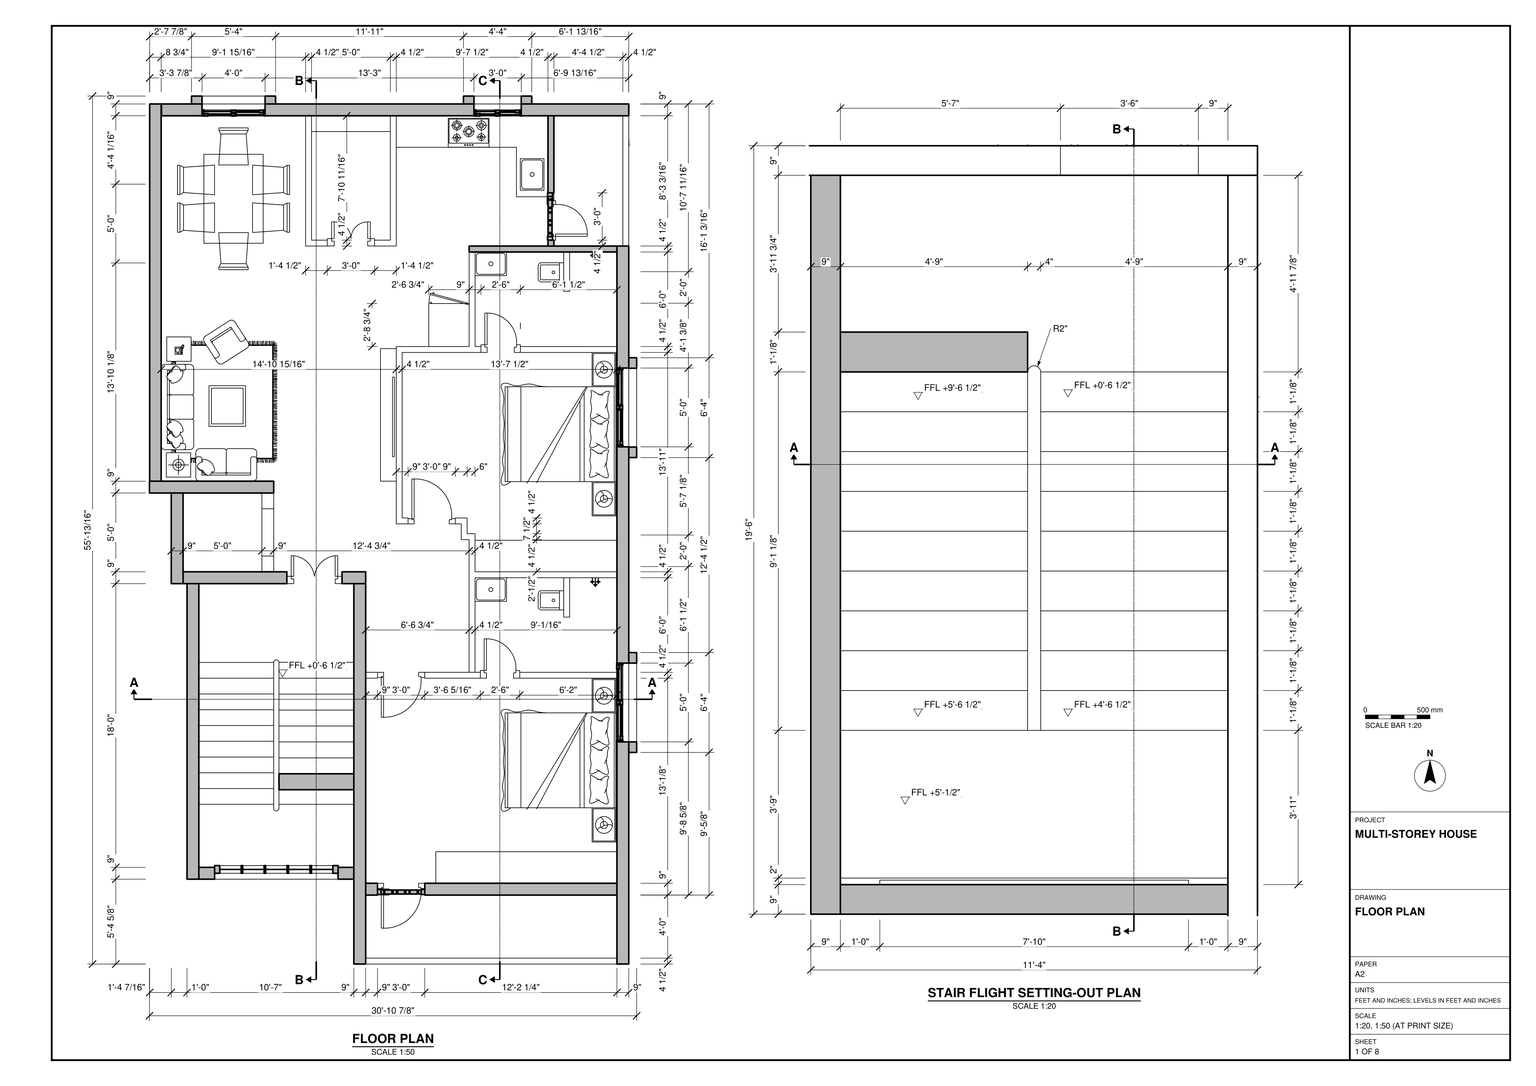
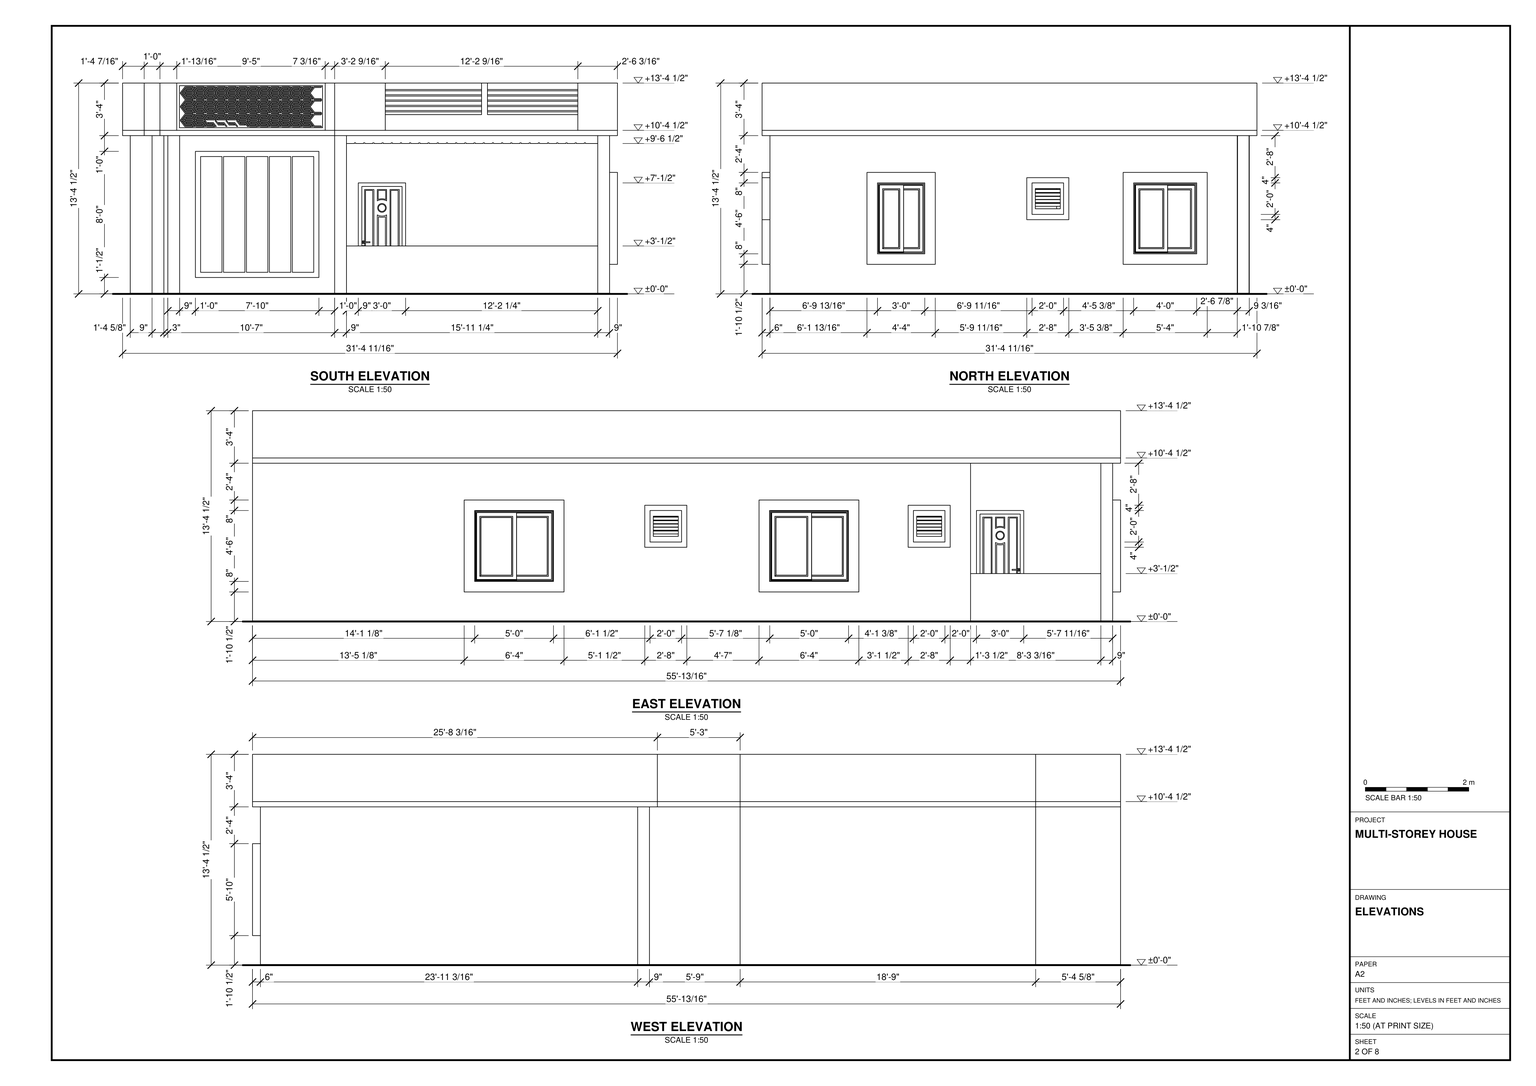
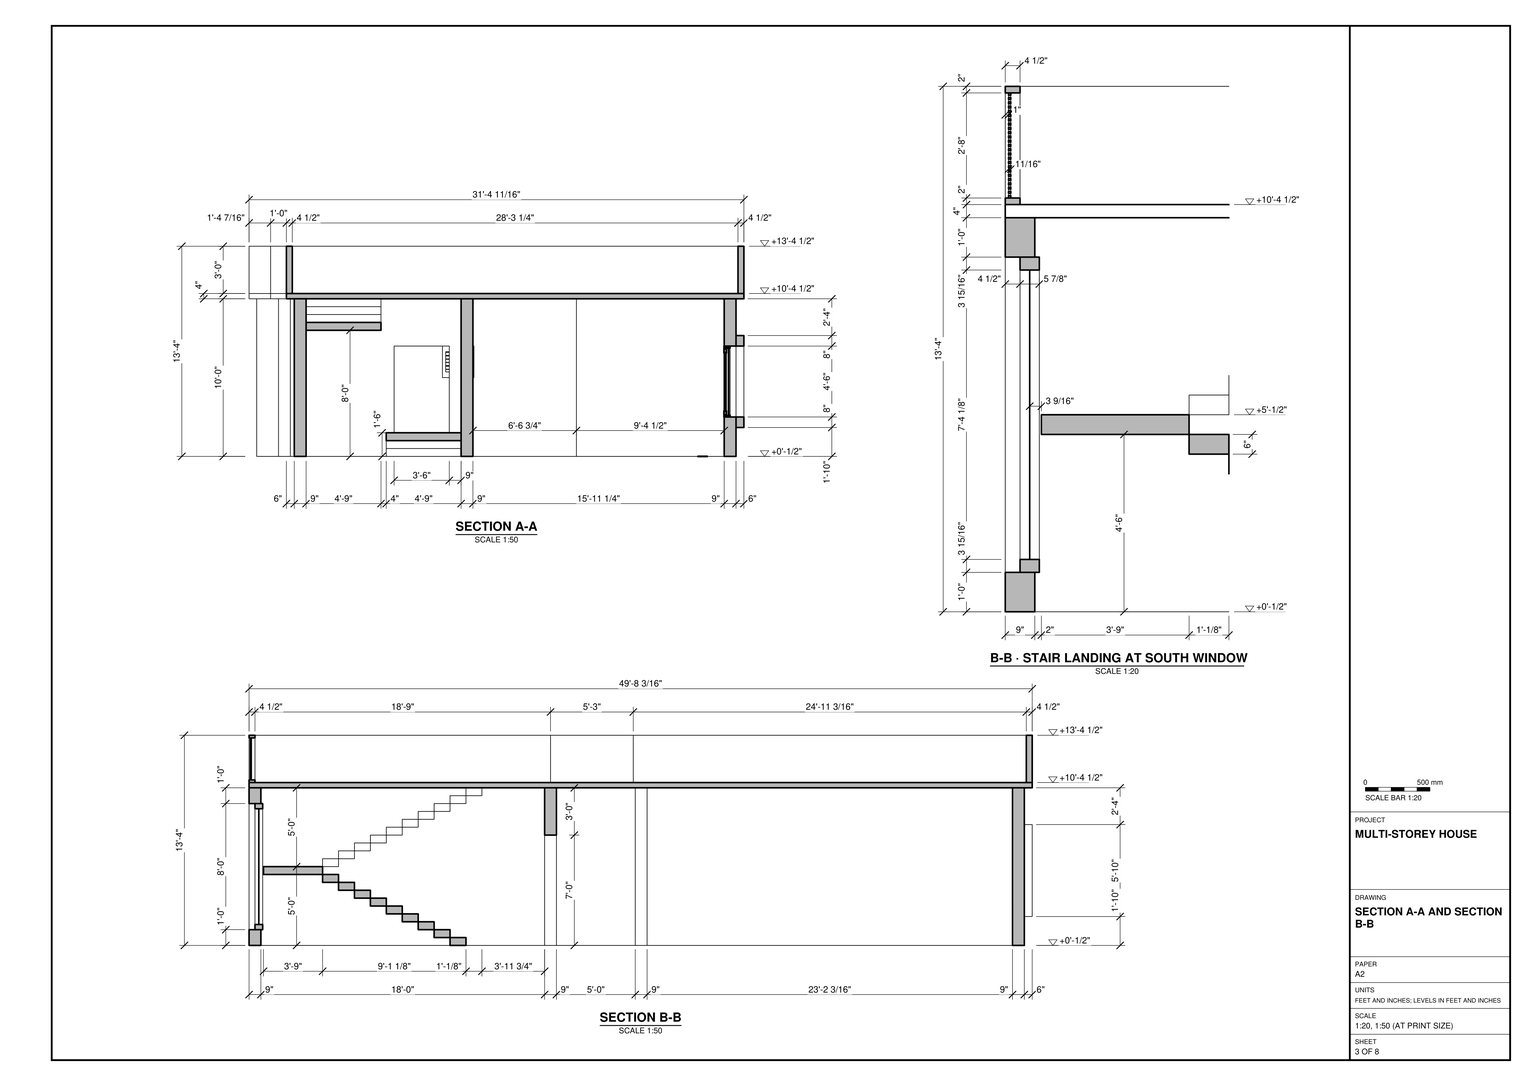
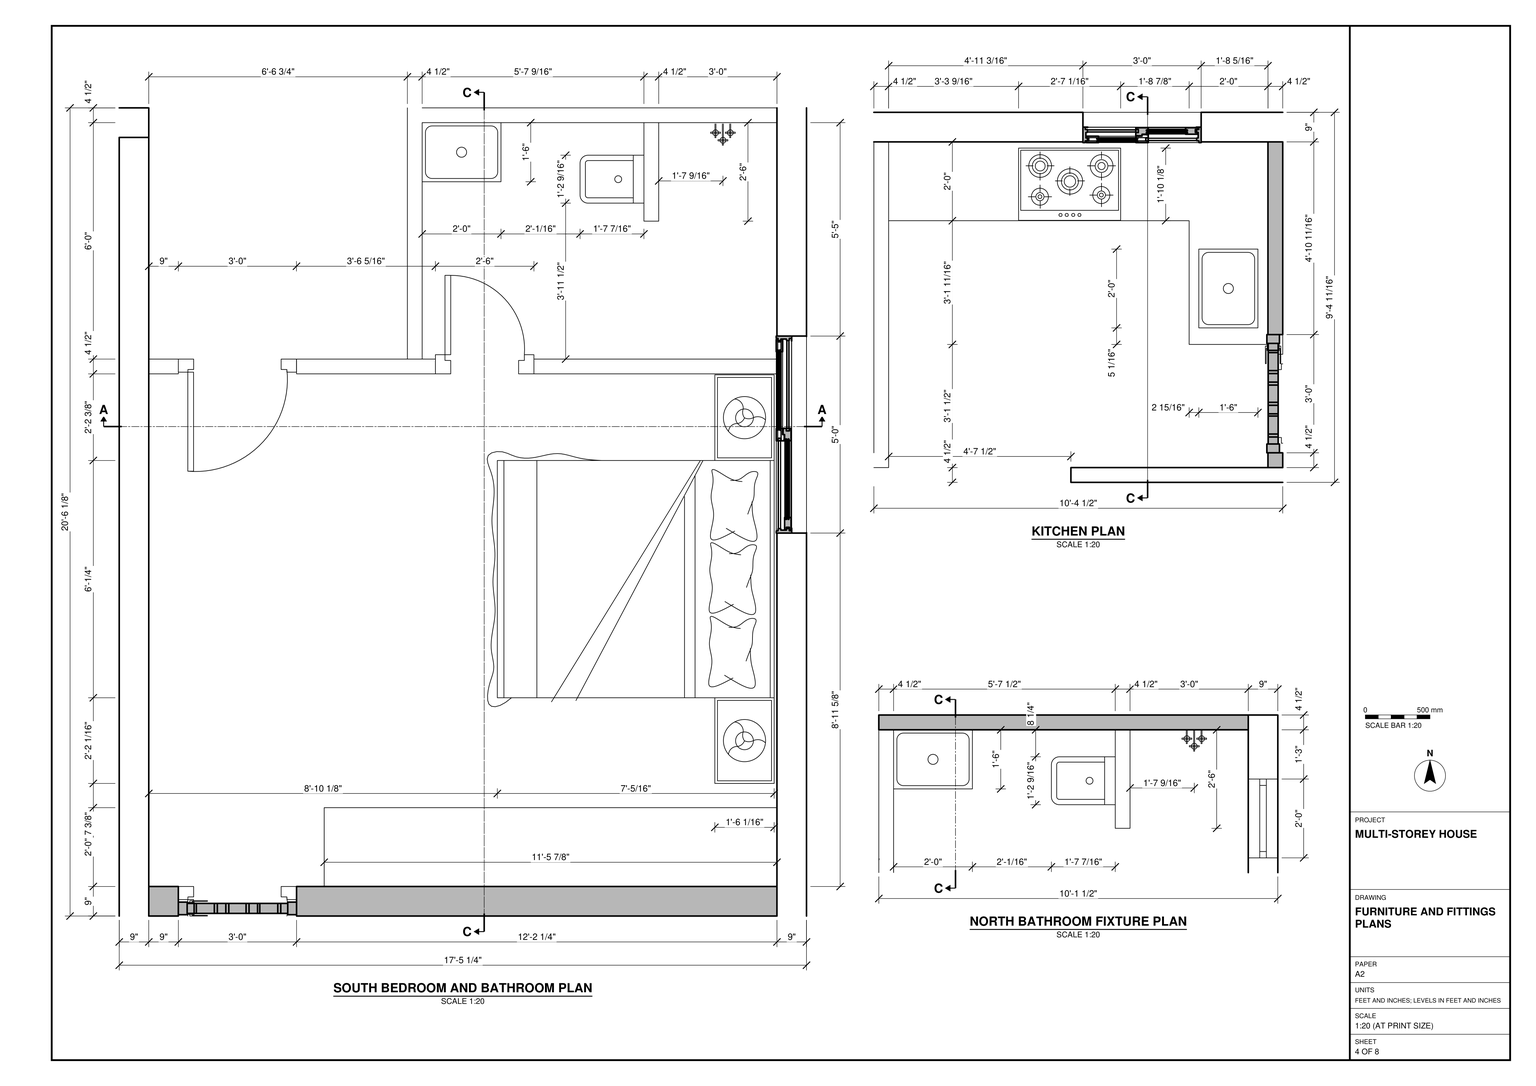
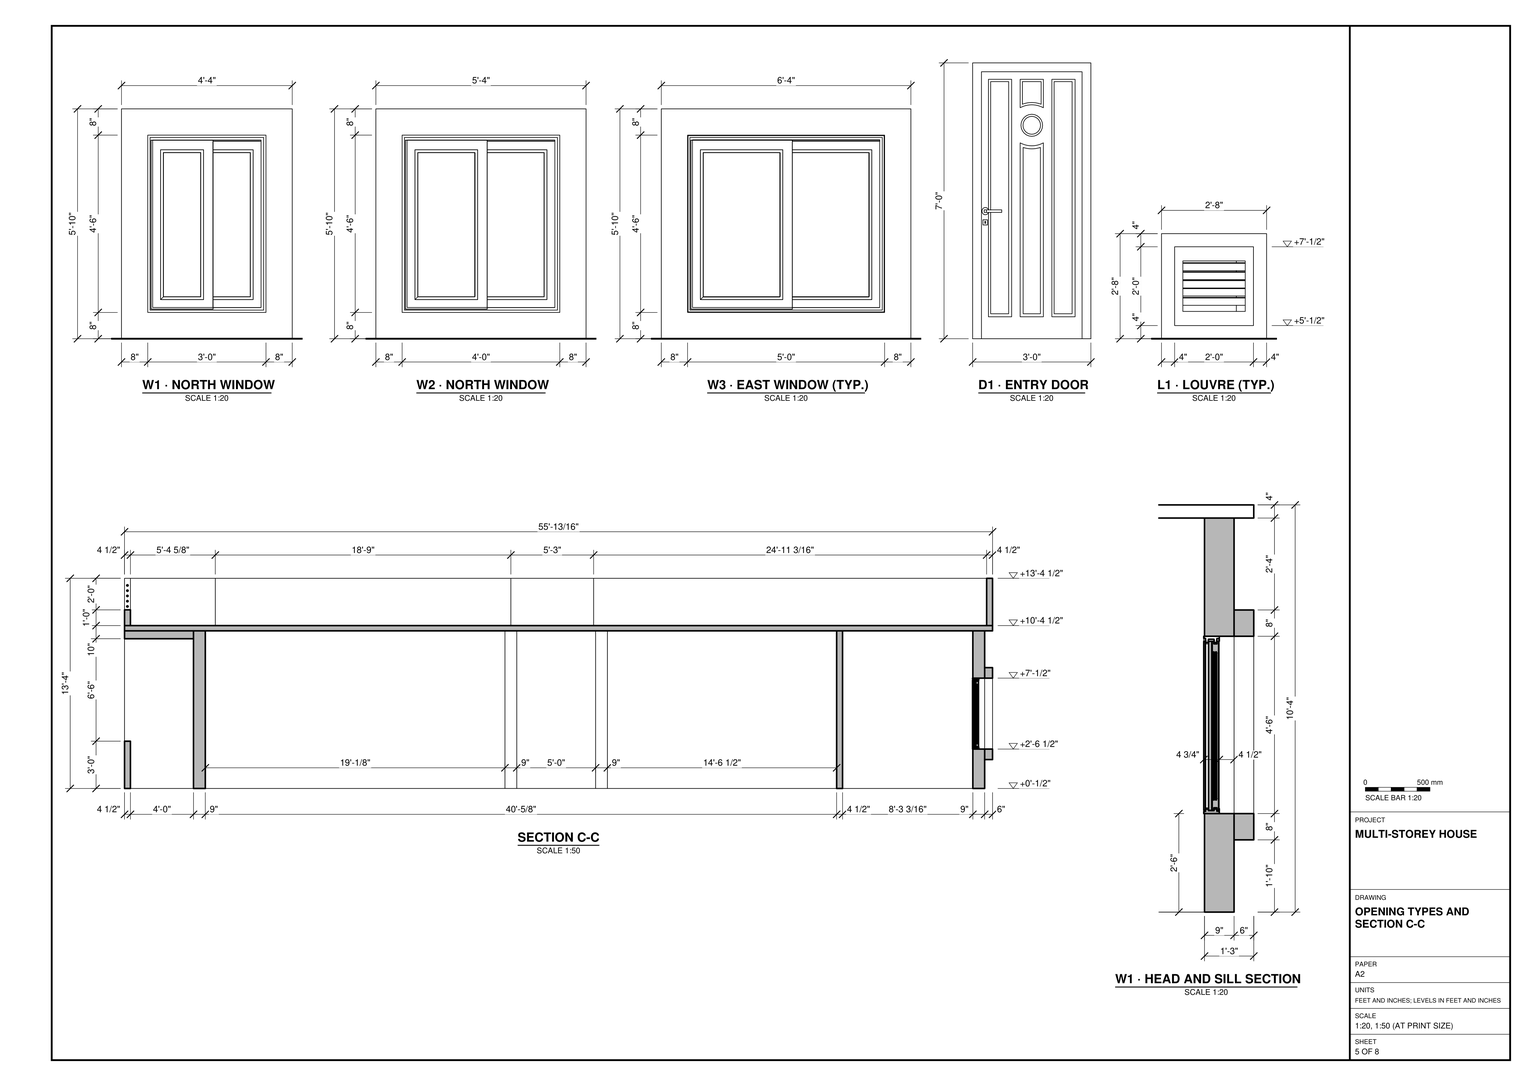
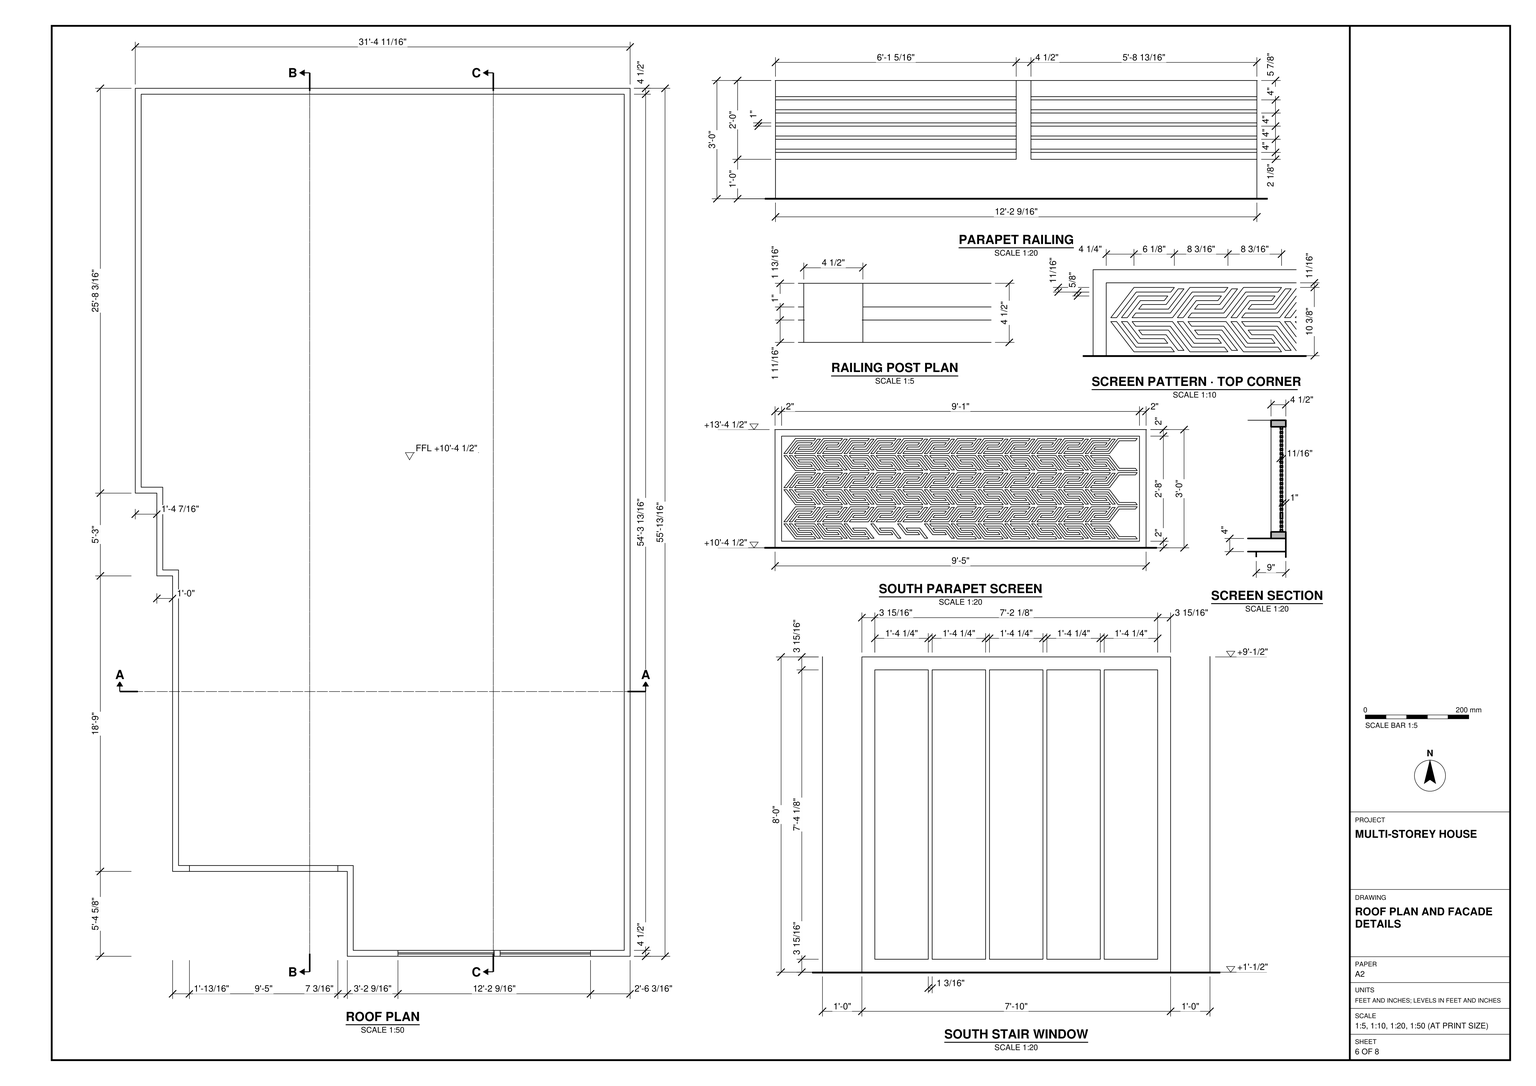
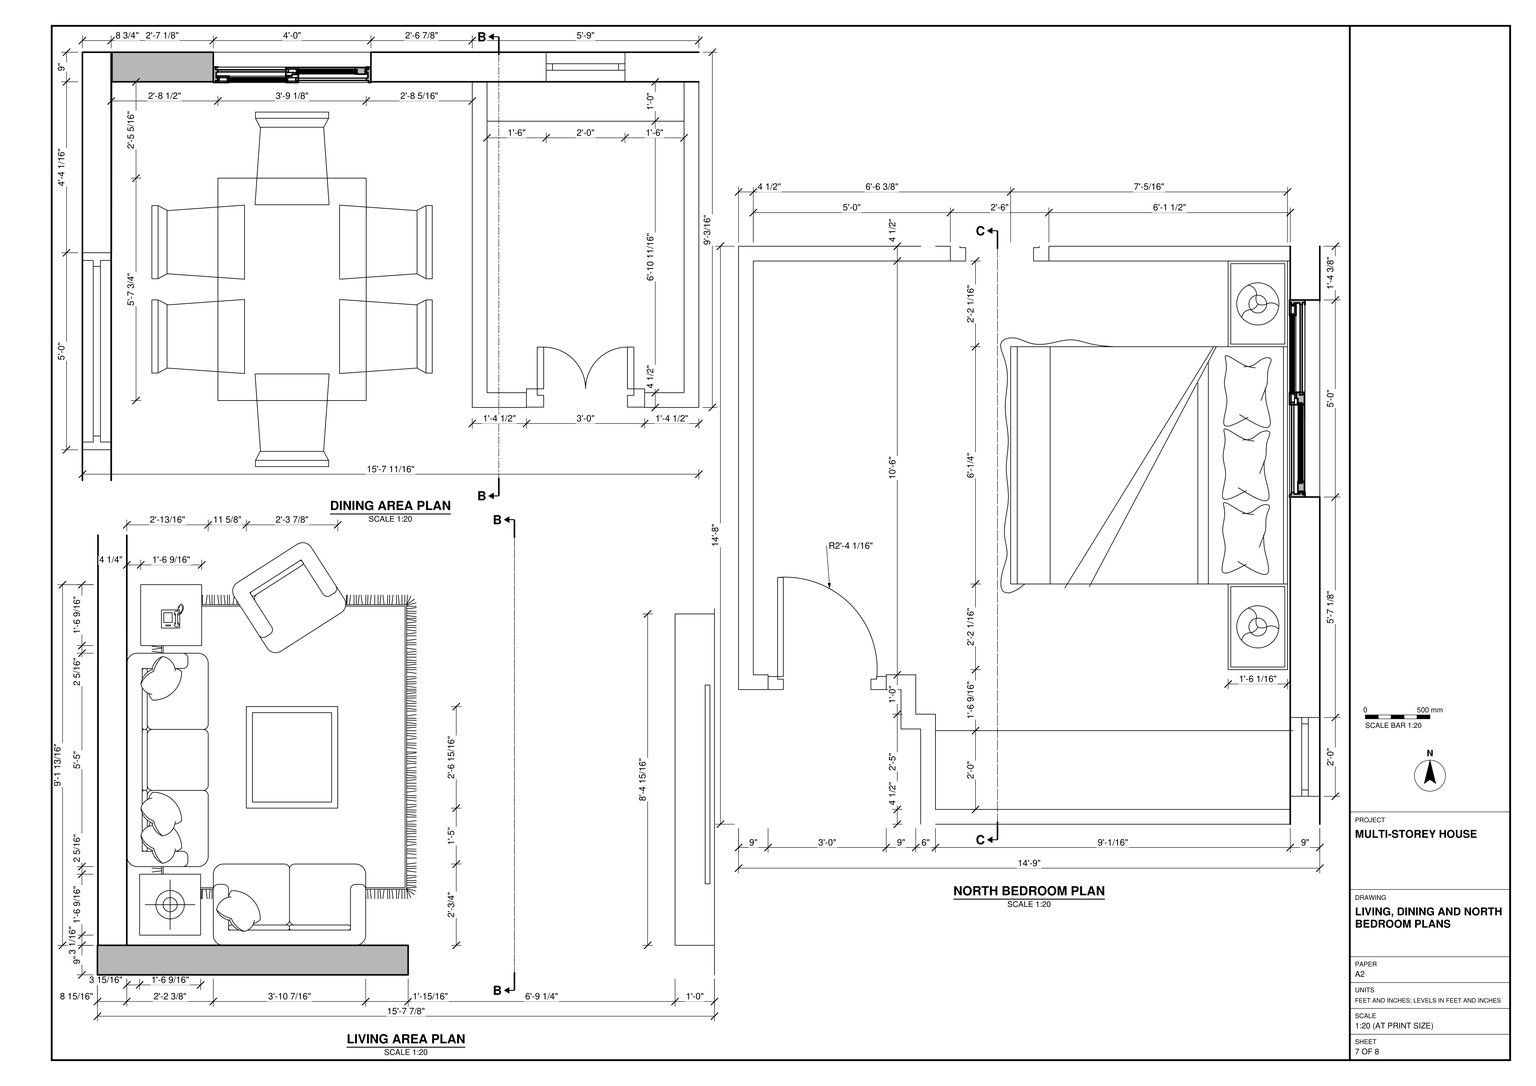
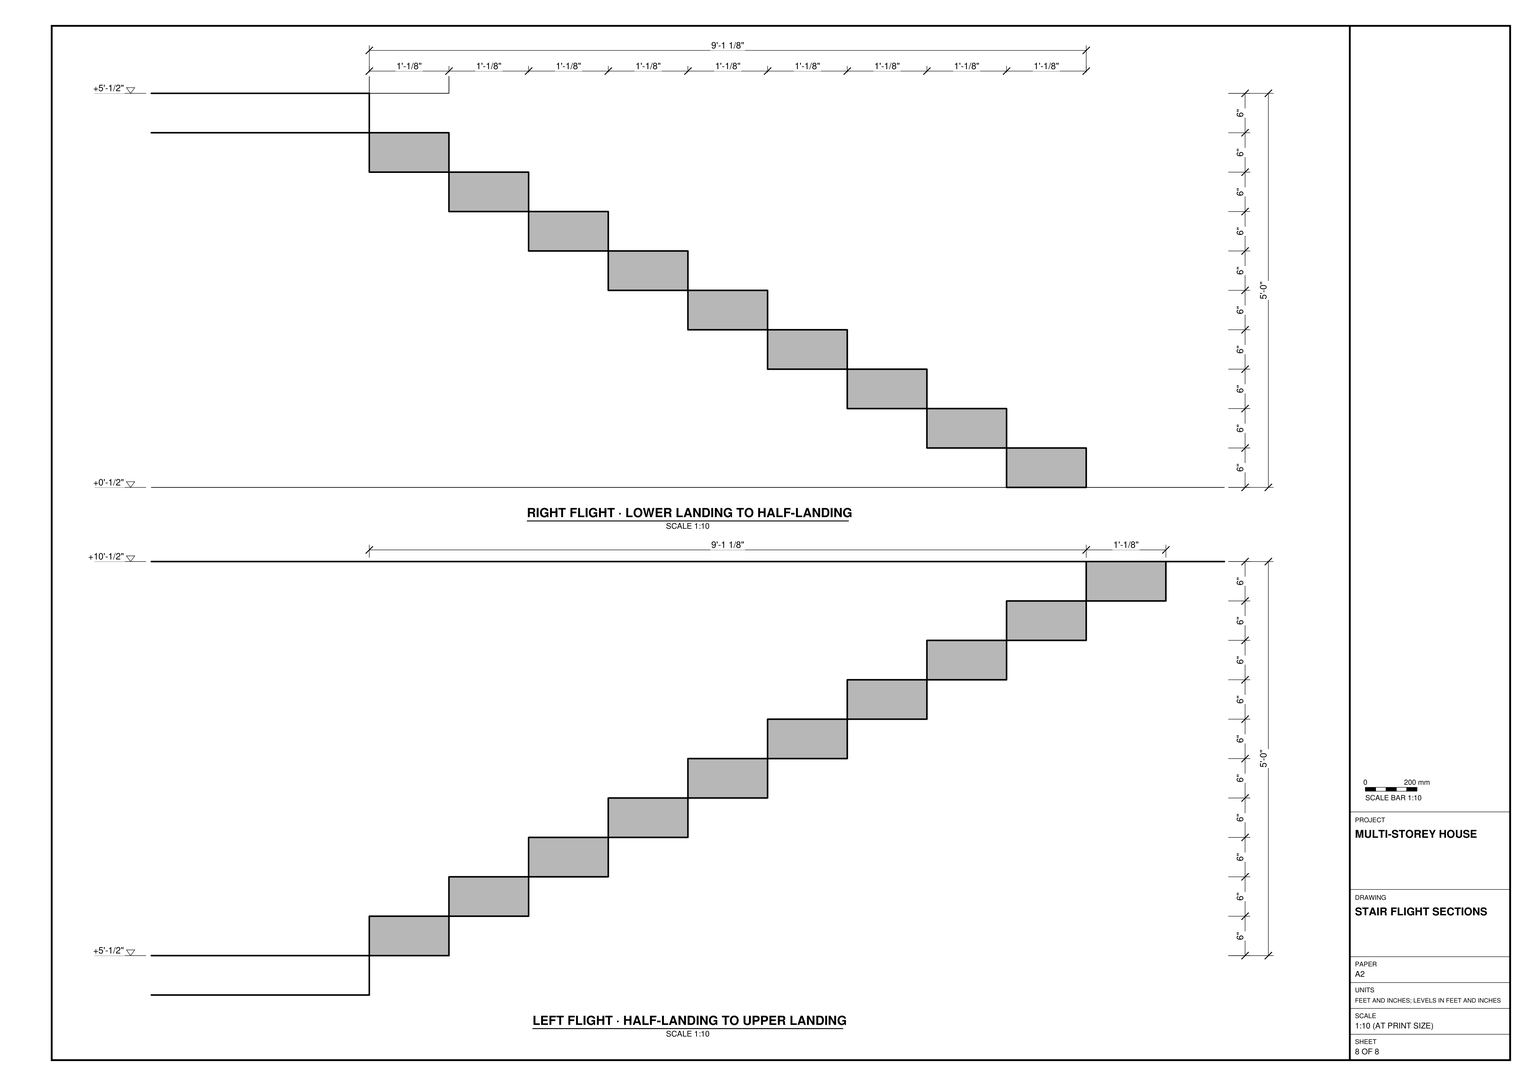
Build the house in SketchUp from task_files/diagram_01.pdf. Work in feet and inches. Set the ground-floor datum to ±0'-0". The overall dimensions, including exterior projections, are 31'-4 11/16" along X, 55'-13/16" along Y and 13'-4 1/2" in height.

Follow the floor plan for the stepped footprint, recessed entrance and room connections. Place the living and dining areas on the west side, the kitchen at the north end and the two bedrooms and adjoining bathrooms along the east side. Use the wall thicknesses shown, distinguishing the 9" walls from the 4 1/2" partitions. Model the floor slab, doors, framed windows and ventilators. Use the stair setting-out plan and sections to build the two parallel flights and their connecting landing at the tall south window. Model the flat roof slab and parapet, including the perforated screen and horizontal slats on the south elevation.

Fit the kitchen counters, sink and cooktop to the plan. Include the bathroom fixtures, beds, bedside tables, living room seating and dining furniture at the sizes and positions drawn. Decor and loose items may be any suitable library components. Keep shell elements such as walls, slabs and roof, and each furniture or joinery piece, as separate groups or components; use components for repeated parts. Save one SketchUp model as output_files/two_bedroom_house_with_a_return_stair_and_flat_roof.skp.

# SketchUp Ruby script. Lengths in inches.
U = 1.inch
M = Sketchup.active_model
def pt(a) = Geom::Point3d.new(a.map { |v| v * U })
def face(e, loops, mat)
  f = e.add_face(loops[0].map { |a| pt(a) })
  loops[1..].each { |l| e.add_face(l.map { |a| pt(a) }).erase! }
  f.material = f.back_material = mat if mat
  f
end
# faces: each face lists its corners as indices into pts; further lists are holes
def faces(e, pts, list, mat = nil) = list.each { |f| face(e, (f[0].is_a?(Array) ? f : [f]).map { |l| l.map { |i| pts[i] } }, mat) }
# xy, xz, yz: faces in a plane at the given z, y or x. An outline is a flat list of corners, or four numbers for a rectangle; further outlines are holes
def ring(l) = l.size == 4 ? [[l[0], l[1]], [l[2], l[1]], [l[2], l[3]], [l[0], l[3]]] : l.each_slice(2).to_a
def flat(e, list, mat, &to3) = list.each { |f| face(e, (f[0].is_a?(Array) ? f : [f]).map { |l| ring(l).map { |u, v| to3.(u, v) } }, mat) }
def xy(e, z, list, mat = nil) = flat(e, list, mat) { |x, y| [x, y, z] }
def xz(e, y, list, mat = nil) = flat(e, list, mat) { |x, z| [x, y, z] }
def yz(e, x, list, mat = nil) = flat(e, list, mat) { |y, z| [x, y, z] }
def lines(e, pts, list) = list.each { |a, b| e.add_line(pt(pts[a]), pt(pts[b])) }
# prism: a flat outline (further loops are holes) pulled along v
def prism(e, loops, v, mat = nil)
  f = face(e, loops, mat); d = Geom::Vector3d.new(v.map { |x| x * U })
  f.pushpull(f.normal.samedirection?(d) ? d.length : -d.length)
end
def box(e, o, s, mat = nil) = prism(e, [[o, [o[0] + s[0], o[1], o[2]], [o[0] + s[0], o[1] + s[1], o[2]], [o[0], o[1] + s[1], o[2]]]], [0, 0, s[2]], mat)
def at(x, y, z, deg = 0) = Geom::Transformation.translation(pt([x, y, z])) * Geom::Transformation.rotation(ORIGIN, Z_AXIS, deg.degrees)
def axes(o, x, y, z) = Geom::Transformation.new([*x, 0, *y, 0, *z, 0, *pt(o).to_a, 1])
def part(name) = M.definitions.add(name)
# library, detail: a bought-in or finely detailed component or shape, given as its bounding box
def library(name, o, s) = part(name).tap { |d| box(d.entities, o, s) }
def detail(e, o, s) = box(e.add_group.entities, o, s)
def put(e, d, t, mat = nil) = e.add_instance(d, t).tap { |i| i.material = mat if mat }
def group(e, t, mat = nil) = e.add_group.tap { |g| g.transformation = t; g.material = mat if mat }.entities
root = M.entities
M.materials.add("E01_Mint_Frost").color = [255, 255, 204]
M.materials.add("Glass_Basic_01").color = [161, 173, 186]
M.materials["Glass_Basic_01"].alpha = 0.25
M.materials.add("M02_Ash_Whisper").color = [196, 196, 196]
M.materials.add("M04_Stone_Frost").color = [142, 142, 142]
M.materials.add("M06_Steel_Smoke").color = [86, 86, 86]
M.materials.add("M07_Charcoal_Gleam").color = [58, 58, 58]
M.materials.add("TEAKcrown-cut").color = [186, 122, 55]
M.materials.add("Wood_Floor_01_1K").color = [146, 111, 76]
M.materials.add("[Translucent_Glass_Gray]3").color = [255, 255, 255]
M.materials["[Translucent_Glass_Gray]3"].alpha = 0.5
c1 = library("PLAN 2BHK.dwg",[2986,411.22,100.3],[365.19,654.78,1])
c2 = library("door58",[0,0,0],[34.0625,4.69,78.29])
c3 = library("AS-120-mm",[0,0,0],[48,4.72,54])
c4 = library("AS-120-mm\#2",[0,0,0],[36,4.72,54])
c5 = library("AS-120-mm\#3",[0,0,0],[60,4.72,54])
c6 = library("JALI+2",[65.125,-1,0],[45.42,1,156.95])
c7 = part("Component\#10")
box(c7.entities,[0,0,0],[19,0.25,3.7],"[Translucent_Glass_Gray]3")
c8 = part("Ventilation_window")
g1 = group(c8.entities,at(-76.91,6.38,0),"TEAKcrown-cut")
xy(g1,-1.7,[[0,0,24,3]])
xy(g1,2.5,[[2.5,0,21.5,3]])
xy(g1,17.5,[[2.5,0,21.5,3]])
xy(g1,21.7,[[0,0,24,3]])
xz(g1,0,[[[0,-1.7,24,21.7],[2.5,2.5,21.5,17.5]]],"TEAKcrown-cut")
xz(g1,3,[[[0,-1.7,24,21.7],[2.5,2.5,21.5,17.5]]])
yz(g1,0,[[0,-1.7,3,21.7]])
yz(g1,2.5,[[0,2.5,3,2.5,3,4.31,0,6.48],[3,4.31,3,17.5,0,17.5,0,6.48]])
yz(g1,21.5,[[0,2.5,3,17.5]])
yz(g1,24,[[0,-1.7,3,21.7]])
put(g1,c7,axes([2.5,3.14,11.94],[1,0,0],[0,0.58779,0.80902],[0,-0.80902,0.58779]))
put(g1,c7,axes([2.5,3.16,14.6],[1,0,0],[0,0.58779,0.80902],[0,-0.80902,0.58779]))
put(g1,c7,axes([2.5,3,4.31],[1,0,0],[0,0.58779,0.80902],[0,-0.80902,0.58779]))
put(g1,c7,axes([2.5,3.14,9.46],[1,0,0],[0,0.58779,0.80902],[0,-0.80902,0.58779]))
put(g1,c7,axes([2.5,2.99,7.08],[1,0,0],[0,0.58779,0.80902],[0,-0.80902,0.58779]))
c9 = part("Group\#16")
box(c9.entities,[0,0,0],[57,12.13,6])
c10 = part("Group94\#2")
xy(c10.entities,0,[[-43.0625,-44.0625,-26.79,44.0625],[-25.6,-44.0625,-9.32,44.0625],[-8.14,-44.0625,8.14,44.0625],[9.32,-44.0625,25.6,44.0625],[26.79,-44.0625,43.0625,44.0625]])
c11 = part("Group93\#1")
prism(c11.entities,[[[47,-48,0],[-47,-48,0],[-47,48,0],[47,48,0]],[[26.79,44.0625,0],[26.79,-44.0625,0],[43.0625,-44.0625,0],[43.0625,44.0625,0]],[[9.32,44.0625,0],[9.32,-44.0625,0],[25.6,-44.0625,0],[25.6,44.0625,0]],[[-43.0625,44.0625,0],[-43.0625,-44.0625,0],[-26.79,-44.0625,0],[-26.79,44.0625,0]],[[-25.6,-44.0625,0],[-9.32,-44.0625,0],[-9.32,44.0625,0],[-25.6,44.0625,0]],[[-8.14,-44.0625,0],[8.14,-44.0625,0],[8.14,44.0625,0],[-8.14,44.0625,0]]],[0,0,5.875])
put(c11.entities,c10,at(0,0,2.9375),"Glass_Basic_01")
c12 = part("Group\#21")
yz(c12.entities,146.58,[[0.47,0,0.6,0.01,0.72,0.05,0.83,0.125,0.92,0.22,0.97,0.34,1,0.47,0.99,0.6,0.95,0.72,0.875,0.83,0.78,0.92,0.66,0.97,0.53,1,0.4,0.99,0.28,0.95,0.17,0.875,0.08,0.78,0.03,0.66,0,0.53,0.01,0.4,0.05,0.28,0.125,0.17,0.22,0.08,0.34,0.03]])
p = [[146.58,0.34,0.03],[146.58,0.22,0.08],[0,0.22,0.08],[0,0.34,0.03],[146.58,0.47,0],[0,0.47,0],
  [146.58,0.6,0.01],[0,0.6,0.01],[146.58,0.72,0.05],[0,0.72,0.05],[146.58,0.125,0.17],[0,0.125,0.17],
  [146.58,0.83,0.125],[0,0.83,0.125],[146.58,0.92,0.22],[0,0.92,0.22],[146.58,0.05,0.28],[0,0.05,0.28],
  [146.58,0.97,0.34],[0,0.97,0.34],[146.58,0.01,0.4],[0,0.01,0.4],[146.58,1,0.47],[0,1,0.47],
  [146.58,0,0.53],[0,0,0.53],[146.58,0.03,0.66],[0,0.03,0.66],[146.58,0.99,0.6],[0,0.99,0.6],
  [146.58,0.95,0.72],[0,0.95,0.72],[146.58,0.08,0.78],[0,0.08,0.78],[146.58,0.875,0.83],[0,0.875,0.83],
  [146.58,0.17,0.875],[0,0.17,0.875],[146.58,0.78,0.92],[0,0.78,0.92],[146.58,0.28,0.95],[0,0.28,0.95],
  [146.58,0.4,0.99],[0,0.4,0.99],[146.58,0.66,0.97],[0,0.66,0.97],[146.58,0.53,1],[0,0.53,1]]
faces(c12.entities,p,[[0,1,2,3],[4,0,3,5],[6,4,5,7],[8,6,7,9],[1,10,11,2],[12,8,9,13],[14,12,13,15],[10,16,17,11],
  [18,14,15,19],[16,20,21,17],[22,18,19,23],[20,24,25,21],[24,26,27,25],[28,22,23,29],[30,28,29,31],[26,32,33,27],
  [34,30,31,35],[32,36,37,33],[38,34,35,39],[36,40,41,37],[40,42,43,41],[44,38,39,45],[42,46,47,43],[46,44,45,47]])
c13 = part("Group\#24")
xy(c13.entities,0,[[0,0,6,76]])
xy(c13.entities,8,[[0,8,6,68]])
xy(c13.entities,62,[[0,8,6,68]])
xy(c13.entities,70,[[0,0,6,76]])
xz(c13.entities,0,[[0,0,6,70]])
xz(c13.entities,8,[[0,8,6,62]])
xz(c13.entities,68,[[0,8,6,62]])
xz(c13.entities,76,[[0,0,6,70]])
yz(c13.entities,0,[[[0,0,76,70],[8,8,68,62]],[[8,8,68,62],[8.15,8.15,67.85,61.85]]])
yz(c13.entities,6,[[[0,0,76,70],[8,8,68,62]]])
c14 = part("Group\#25")
prism(c14.entities,[[[0,0,0],[0,0,32],[0,32,32],[0,32,0]],[[0,4,4],[0,28,4],[0,28,28],[0,4,28]]],[6,0,0])
p = [[55.43,64.6,12],[55.43,64.6,108],[149.43,64.6,108],[149.43,64.6,12]]
lines(root,p,[[0,1],[1,2],[2,3],[3,0]])
put(root,c1,at(-2980.18,-411.22,-100.8))
put(root,c2,axes([179.43,52.5,0],[1.05686,0,0],[0,1,0],[0,0,1.07289]))
put(root,c3,at(45.85,645.5625,30))
put(root,c4,at(252.87,645.5625,30))
put(root,c5,at(361.48,453.74,30,-90))
put(root,c5,at(361.48,229.11,30,-90))
put(root,c6,axes([152.22,66.29,80.125],[0,0,0.70439],[0,0.6844,0],[-0.69434,0,0]))
put(root,c8,axes([376.01,379.52,61.74],[0,1,0],[-1.1457,0,0],[0,0,1.02564]))
put(root,c8,axes([376.01,580.02,61.74],[0,1,0],[-1.1457,0,0],[0,0,1.02564]))
put(root,c8,axes([94.3,660.09,61.74],[-1,0,0],[0,-1.1457,0],[0,0,1.02564]))
put(root,c2,axes([313.12,587.1,0],[0,-1.05686,0],[-1,0,0],[0,0,1.07289]))
g2 = group(root,at(6,367.6,0))
box(g2,[0,0,0],[8.75,287.18,120])
g3 = group(root,at(5.82,358.6,0))
box(g3,[0,0,0],[94.61,9,120])
g4 = group(root,at(22.43,289.6,0))
box(g4,[0,0,0],[9,69,120])
g5 = group(root,at(31.43,289.6,0))
prism(g5,[[[0,0,0],[79,0,0],[79,0,84],[121,0,84],[121,0,0],[139,0,0],[139,0,120],[0,0,120]]],[0,9,0])
g6 = group(root,at(34.43,64.6,0))
xy(g6,0,[[0,0,9,225]])
xy(g6,120,[[0,0,9,225]])
xz(g6,0,[[0,0,9,120]],"E01_Mint_Frost")
xz(g6,225,[[0,0,9,120]])
yz(g6,0,[[0,0,225,120]])
yz(g6,9,[[0,0,225,120]])
g7 = group(root,at(43.43,64.6,0))
xy(g7,0,[[0,0,118,9]])
xy(g7,12,[[12,0,106,9]])
xy(g7,108,[[12,0,106,9]])
xy(g7,120,[[0,0,118,9]],"E01_Mint_Frost")
xz(g7,0,[[[0,0,118,120],[12,12,106,108]]],"E01_Mint_Frost")
xz(g7,9,[[[0,0,118,120],[12,12,106,108]]])
yz(g7,0,[[0,0,9,120]])
yz(g7,12,[[0,12,9,108]])
yz(g7,106,[[0,12,9,108]])
yz(g7,118,[[0,0,9,120]])
g8 = group(root,at(161.43,0,0))
xy(g8,0,[[0,0,9,289.6]])
xy(g8,120,[[0,0,9,289.6]])
xz(g8,0,[[0,0,9,120]],"M04_Stone_Frost")
xz(g8,289.6,[[0,0,9,120]])
yz(g8,0,[[0,0,289.6,120]])
yz(g8,9,[[0,0,289.6,120]])
g9 = group(root,at(170.43,52.5,0))
xy(g9,0,[[0,0,9,9],[45,0,191.28,9]])
xy(g9,84,[[9,0,45,9]])
xy(g9,120,[[0,0,191.28,9]])
xz(g9,0,[[0,0,9,0,9,84,45,84,45,0,191.28,0,191.28,120,0,120]],"M02_Ash_Whisper")
xz(g9,9,[[0,0,0,120,191.28,120,191.28,0,45,0,45,84,9,84,9,0]])
yz(g9,0,[[0,0,9,120]])
yz(g9,9,[[0,0,9,84]])
yz(g9,45,[[0,0,9,84]])
yz(g9,191.28,[[0,0,9,120]])
g10 = group(root,at(361.71,0,0))
xy(g10,0,[[0,0,9,546.6]])
xy(g10,30,[[0,169.11,9,229.11],[0,393.74,9,453.74]])
xy(g10,60,[[0,302.6,9,326.6],[0,503.1,9,527.1]])
xy(g10,84,[[0,169.11,9,229.11],[0,302.6,9,326.6],[0,393.74,9,453.74],[0,503.1,9,527.1]])
xy(g10,120,[[0,0,9,546.6]])
xz(g10,0,[[0,0,9,120]],"M04_Stone_Frost")
xz(g10,169.11,[[0,30,9,84]])
xz(g10,229.11,[[0,30,9,84]])
xz(g10,302.6,[[0,60,9,84]])
xz(g10,326.6,[[0,60,9,84]])
xz(g10,393.74,[[0,30,9,84]])
xz(g10,453.74,[[0,30,9,84]])
xz(g10,503.1,[[0,60,9,84]])
xz(g10,527.1,[[0,60,9,84]])
xz(g10,546.6,[[0,0,9,120]])
yz(g10,0,[[[0,0,546.6,120],[169.11,30,229.11,84],[393.74,30,453.74,84],[503.1,60,527.1,84],[302.6,60,326.6,84]]])
yz(g10,9,[[[0,0,546.6,120],[169.11,30,229.11,84],[393.74,30,453.74,84],[503.1,60,527.1,84],[302.6,60,326.6,84]]])
g11 = group(root,at(249.21,542.1,0))
box(g11,[0,0,0],[112.5,4.5,120])
g12 = group(root,at(309.21,546.6,0))
prism(g12,[[[4.5,0,0],[4.5,4.5,0],[4.5,4.5,84],[4.5,40.5,84],[4.5,40.5,0],[4.5,99.18,0],[4.5,99.18,120],[4.5,0,120]]],[-4.5,0,0])
g13 = group(root,at(14.99,645.79,0))
prism(g13,[[[0,0,0],[355.72,0,0],[355.72,0,120],[0,0,120]],[[78.86,0,30],[30.86,0,30],[30.86,0,84],[78.86,0,84]],[[237.875,0,84],[273.875,0,84],[273.875,0,30],[237.875,0,30]],[[132.22,0,84],[156.22,0,84],[156.22,0,60],[132.22,0,60]]],[0,9,0])
g14 = group(root,at(366.21,546.6,0))
box(g14,[0,0,0],[4.5,99.18,36])
g15 = group(root,at(170.43,0,0),"M04_Stone_Frost")
box(g15,[0,0,0],[191.28,4.5,36])
g16 = group(root,at(43.42,73.6,0))
put(g16,c9,at(61,59.1,42))
put(g16,c9,at(61,83.36,30))
put(g16,c9,at(61,144,0))
put(g16,c9,at(61,107.62,18))
put(g16,c9,at(61,95.49,24))
put(g16,c9,at(61,71.23,36))
put(g16,c9,at(61,46.97,48))
put(g16,c9,at(61,131.87,6))
put(g16,c9,at(0,46.97,60))
put(g16,c9,at(61,119.74,12))
g17 = group(g16,at(61,34.85,54))
box(g17,[-61,-32.85,0],[118,44.98,6])
put(g16,c9,at(0,71.23,72))
put(g16,c9,at(0,131.87,102))
put(g16,c9,at(0,144,108))
put(g16,c9,at(0,156.13,114))
put(g16,c9,at(0,107.62,90))
put(g16,c9,at(0,59.1,66))
put(g16,c9,at(0,83.36,78))
put(g16,c9,at(0,95.49,84))
put(g16,c9,at(0,119.74,96))
g18 = group(root,at(0,0,120))
xy(g18,0,[[161.43,0,161.43,64.6,28.43,64.6,28.43,289.6,16.43,289.6,16.43,352.6,0,352.6,0,660.79,376.71,660.79,376.71,0]],"M04_Stone_Frost")
xy(g18,4,[[161.43,0,376.71,0,376.71,660.79,0,660.79,0,352.6,16.43,352.6,16.43,289.6,28.43,289.6,28.43,64.6,161.43,64.6]])
xz(g18,0,[[161.43,0,376.71,4]],"M04_Stone_Frost")
xz(g18,64.6,[[28.43,0,161.43,4]])
xz(g18,289.6,[[16.43,0,28.43,4]])
xz(g18,352.6,[[0,0,16.43,4]])
xz(g18,660.79,[[0,0,376.71,4]])
yz(g18,0,[[352.6,0,660.79,4]])
yz(g18,16.43,[[289.6,0,352.6,4]])
yz(g18,28.43,[[64.6,0,289.6,4]])
yz(g18,161.43,[[0,0,64.6,4]])
yz(g18,376.71,[[0,0,660.79,4]])
g19 = group(root,at(0,0,124))
xy(g19,0,[[[161.43,0,161.43,64.6,28.43,64.6,28.43,289.6,16.43,289.6,16.43,352.6,0,352.6,0,660.79,376.71,660.79,376.71,0],[165.93,4.5,372.21,4.5,372.21,656.29,4.5,656.29,4.5,357.1,20.93,357.1,20.93,294.1,32.93,294.1,32.93,69.1,165.93,69.1]]])
xy(g19,2,[[43.24,64.6,152.22,69.1]])
xy(g19,12,[[199.97,0,273.26,4.5],[277.76,0,346.55,4.5]],"M04_Stone_Frost")
xy(g19,34,[[43.24,64.6,152.22,69.1]])
xy(g19,36,[[346.55,0,376.71,0,376.71,660.79,0,660.79,0,352.6,16.43,352.6,16.43,289.6,28.43,289.6,28.43,64.6,41.24,64.6,41.24,69.1,32.93,69.1,32.93,294.1,20.93,294.1,20.93,357.1,4.5,357.1,4.5,656.29,372.21,656.29,372.21,4.5,346.55,4.5],[161.43,0,199.97,0,199.97,4.5,165.93,4.5,165.93,69.1,154.22,69.1,154.22,64.6,161.43,64.6],[41.24,64.6,154.22,69.1]])
xy(g19,36,[[273.26,0,277.76,4.5]],"M04_Stone_Frost")
xz(g19,0,[[161.43,0,199.97,36],[199.97,0,346.55,0,346.55,12,277.76,12,277.76,36,273.26,36,273.26,12,199.97,12],[346.55,0,376.71,36]],"M04_Stone_Frost")
xz(g19,4.5,[[165.93,0,165.93,36,199.97,36,199.97,12,273.26,12,273.26,36,277.76,36,277.76,12,346.55,12,346.55,36,372.21,36,372.21,0]])
xz(g19,64.6,[[28.43,0,41.24,36],[[41.24,0,154.22,36],[43.24,2,152.22,34]],[154.22,0,161.43,36]],"E01_Mint_Frost")
xz(g19,69.1,[[[32.93,0,165.93,36],[43.24,2,152.22,34]]])
xz(g19,289.6,[[16.43,0,28.43,36]])
xz(g19,294.1,[[20.93,0,32.93,36]])
xz(g19,352.6,[[0,0,16.43,36]])
xz(g19,357.1,[[4.5,0,20.93,36]])
xz(g19,656.29,[[4.5,0,372.21,36]])
xz(g19,660.79,[[0,0,376.71,36]])
yz(g19,0,[[352.6,0,660.79,36]])
yz(g19,4.5,[[357.1,0,656.29,36]])
yz(g19,16.43,[[289.6,0,352.6,36]])
yz(g19,20.93,[[294.1,0,357.1,36]])
yz(g19,28.43,[[64.6,0,289.6,36]])
yz(g19,32.93,[[69.1,0,294.1,36]])
yz(g19,43.24,[[64.6,2,69.1,34]])
yz(g19,152.22,[[64.6,2,69.1,34]])
yz(g19,161.43,[[0,0,64.6,36]])
yz(g19,165.93,[[4.5,0,69.1,36]])
yz(g19,199.97,[[0,12,4.5,36]])
yz(g19,273.26,[[0,12,4.5,36]])
yz(g19,277.76,[[0,12,4.5,36]],"M04_Stone_Frost")
yz(g19,346.55,[[0,12,4.5,36]])
yz(g19,372.21,[[4.5,0,656.29,36]])
yz(g19,376.71,[[0,0,660.79,36]])
put(root,c11,axes([102.43,74.98,60],[1,0,0],[0,0,1],[0,-1,0]),"M07_Charcoal_Gleam")
put(root,c12,at(199.97,1.7,138.1),"M06_Steel_Smoke")
put(root,c12,at(199.97,1.7,142.1),"M06_Steel_Smoke")
put(root,c12,at(199.97,1.7,146.1),"M06_Steel_Smoke")
put(root,c12,at(199.97,1.7,150.1),"M06_Steel_Smoke")
put(root,c12,at(199.97,1.7,154.1),"M06_Steel_Smoke")
g20 = group(root,at(170.43,0,114))
xy(g20,0,[[188,0,191.28,52.5]])
xy(g20,0,[[0,0,6,52.5],[7,0,13,52.5],[14,0,20,52.5],[21,0,27,52.5],[28,0,34,52.5],
  [35,0,41,52.5],[42,0,48,52.5],[49,0,55,52.5],[56,0,62,52.5],[63,0,69,52.5],
  [70,0,76,52.5],[77,0,83,52.5],[84,0,90,52.5],[91,0,97,52.5],[98,0,104,52.5],
  [105,0,111,52.5],[112,0,118,52.5],[119,0,125,52.5],[126,0,132,52.5],[133,0,139,52.5],
  [140,0,146,52.5],[147,0,153,52.5],[154,0,160,52.5],[161,0,167,52.5],[168,0,174,52.5],
  [175,0,181,52.5],[182,0,188,52.5]],"Wood_Floor_01_1K")
xy(g20,0.5,[[6,0,7,52.5],[13,0,14,52.5],[20,0,21,52.5],[27,0,28,52.5],[34,0,35,52.5],
  [41,0,42,52.5],[48,0,49,52.5],[55,0,56,52.5],[62,0,63,52.5],[69,0,70,52.5],
  [76,0,77,52.5],[83,0,84,52.5],[90,0,91,52.5],[97,0,98,52.5],[104,0,105,52.5],
  [111,0,112,52.5],[118,0,119,52.5],[125,0,126,52.5],[132,0,133,52.5],[139,0,140,52.5],
  [146,0,147,52.5],[153,0,154,52.5],[160,0,161,52.5],[167,0,168,52.5],[174,0,175,52.5],
  [181,0,182,52.5]])
xy(g20,6,[[0,0,191.28,52.5]])
xz(g20,0,[[0,0,6,0,6,0.5,7,0.5,7,0,13,0,13,0.5,14,0.5,14,0,20,0,20,0.5,21,0.5,21,0,27,0,27,0.5,28,0.5,28,0,34,0,34,0.5,35,0.5,35,0,41,0,41,0.5,42,0.5,42,0,48,0,48,0.5,49,0.5,49,0,55,0,55,0.5,56,0.5,56,0,62,0,62,0.5,63,0.5,63,0,69,0,69,0.5,70,0.5,70,0,76,0,76,0.5,77,0.5,77,0,83,0,83,0.5,84,0.5,84,0,90,0,90,0.5,91,0.5,91,0,97,0,97,0.5,98,0.5,98,0,104,0,104,0.5,105,0.5,105,0,111,0,111,0.5,112,0.5,112,0,118,0,118,0.5,119,0.5,119,0,125,0,125,0.5,126,0.5,126,0,132,0,132,0.5,133,0.5,133,0,139,0,139,0.5,140,0.5,140,0,146,0,146,0.5,147,0.5,147,0,153,0,153,0.5,154,0.5,154,0,160,0,160,0.5,161,0.5,161,0,167,0,167,0.5,168,0.5,168,0,174,0,174,0.5,175,0.5,175,0,181,0,181,0.5,182,0.5,182,0,191.28,0,191.28,6,0,6]],"Wood_Floor_01_1K")
xz(g20,52.5,[[0,0,0,6,191.28,6,191.28,0,182,0,182,0.5,181,0.5,181,0,175,0,175,0.5,174,0.5,174,0,168,0,168,0.5,167,0.5,167,0,161,0,161,0.5,160,0.5,160,0,154,0,154,0.5,153,0.5,153,0,147,0,147,0.5,146,0.5,146,0,140,0,140,0.5,139,0.5,139,0,133,0,133,0.5,132,0.5,132,0,126,0,126,0.5,125,0.5,125,0,119,0,119,0.5,118,0.5,118,0,112,0,112,0.5,111,0.5,111,0,105,0,105,0.5,104,0.5,104,0,98,0,98,0.5,97,0.5,97,0,91,0,91,0.5,90,0.5,90,0,84,0,84,0.5,83,0.5,83,0,77,0,77,0.5,76,0.5,76,0,70,0,70,0.5,69,0.5,69,0,63,0,63,0.5,62,0.5,62,0,56,0,56,0.5,55,0.5,55,0,49,0,49,0.5,48,0.5,48,0,42,0,42,0.5,41,0.5,41,0,35,0,35,0.5,34,0.5,34,0,28,0,28,0.5,27,0.5,27,0,21,0,21,0.5,20,0.5,20,0,14,0,14,0.5,13,0.5,13,0,7,0,7,0.5,6,0.5,6,0]])
yz(g20,0,[[0,0,52.5,6]])
yz(g20,6,[[0,0,52.5,0.5]])
yz(g20,7,[[0,0,52.5,0.5]])
yz(g20,13,[[0,0,52.5,0.5]])
yz(g20,14,[[0,0,52.5,0.5]])
yz(g20,20,[[0,0,52.5,0.5]])
yz(g20,21,[[0,0,52.5,0.5]])
yz(g20,27,[[0,0,52.5,0.5]])
yz(g20,28,[[0,0,52.5,0.5]])
yz(g20,34,[[0,0,52.5,0.5]])
yz(g20,35,[[0,0,52.5,0.5]])
yz(g20,41,[[0,0,52.5,0.5]])
yz(g20,42,[[0,0,52.5,0.5]])
yz(g20,48,[[0,0,52.5,0.5]])
yz(g20,49,[[0,0,52.5,0.5]])
yz(g20,55,[[0,0,52.5,0.5]])
yz(g20,56,[[0,0,52.5,0.5]])
yz(g20,62,[[0,0,52.5,0.5]])
yz(g20,63,[[0,0,52.5,0.5]])
yz(g20,69,[[0,0,52.5,0.5]])
yz(g20,70,[[0,0,52.5,0.5]])
yz(g20,76,[[0,0,52.5,0.5]])
yz(g20,77,[[0,0,52.5,0.5]])
yz(g20,83,[[0,0,52.5,0.5]])
yz(g20,84,[[0,0,52.5,0.5]])
yz(g20,90,[[0,0,52.5,0.5]])
yz(g20,91,[[0,0,52.5,0.5]])
yz(g20,97,[[0,0,52.5,0.5]])
yz(g20,98,[[0,0,52.5,0.5]])
yz(g20,104,[[0,0,52.5,0.5]])
yz(g20,105,[[0,0,52.5,0.5]])
yz(g20,111,[[0,0,52.5,0.5]])
yz(g20,112,[[0,0,52.5,0.5]])
yz(g20,118,[[0,0,52.5,0.5]])
yz(g20,119,[[0,0,52.5,0.5]])
yz(g20,125,[[0,0,52.5,0.5]])
yz(g20,126,[[0,0,52.5,0.5]])
yz(g20,132,[[0,0,52.5,0.5]])
yz(g20,133,[[0,0,52.5,0.5]])
yz(g20,139,[[0,0,52.5,0.5]])
yz(g20,140,[[0,0,52.5,0.5]])
yz(g20,146,[[0,0,52.5,0.5]])
yz(g20,147,[[0,0,52.5,0.5]])
yz(g20,153,[[0,0,52.5,0.5]])
yz(g20,154,[[0,0,52.5,0.5]])
yz(g20,160,[[0,0,52.5,0.5]])
yz(g20,161,[[0,0,52.5,0.5]])
yz(g20,167,[[0,0,52.5,0.5]])
yz(g20,168,[[0,0,52.5,0.5]])
yz(g20,174,[[0,0,52.5,0.5]])
yz(g20,175,[[0,0,52.5,0.5]])
yz(g20,181,[[0,0,52.5,0.5]])
yz(g20,182,[[0,0,52.5,0.5]])
yz(g20,191.28,[[0,0,52.5,6]])
put(root,c13,at(370.71,161.11,22),"M04_Stone_Frost")
put(root,c13,at(370.71,385.59,22),"M04_Stone_Frost")
put(root,c14,at(370.71,298.6,56),"M04_Stone_Frost")
put(root,c14,at(370.71,499.1,56),"M04_Stone_Frost")
g21 = group(root,at(244.87,654.79,22),"M04_Stone_Frost")
prism(g21,[[[0,6,0],[0,6,70],[52,6,70],[52,6,0]],[[44,6,62],[8,6,62],[8,6,8],[44,6,8]]],[0,-6,0])
g22 = group(root,at(37.85,654.79,22),"M04_Stone_Frost")
prism(g22,[[[0,6,70],[64,6,70],[64,6,0],[0,6,0]],[[56,6,8],[56,6,62],[8,6,62],[8,6,8]]],[0,-6,0])
g23 = group(root,at(143.21,654.79,56),"M04_Stone_Frost")
prism(g23,[[[32,6,32],[32,6,0],[0,6,0],[0,6,32]],[[28,6,4],[28,6,28],[4,6,28],[4,6,4]]],[0,-6,0])
